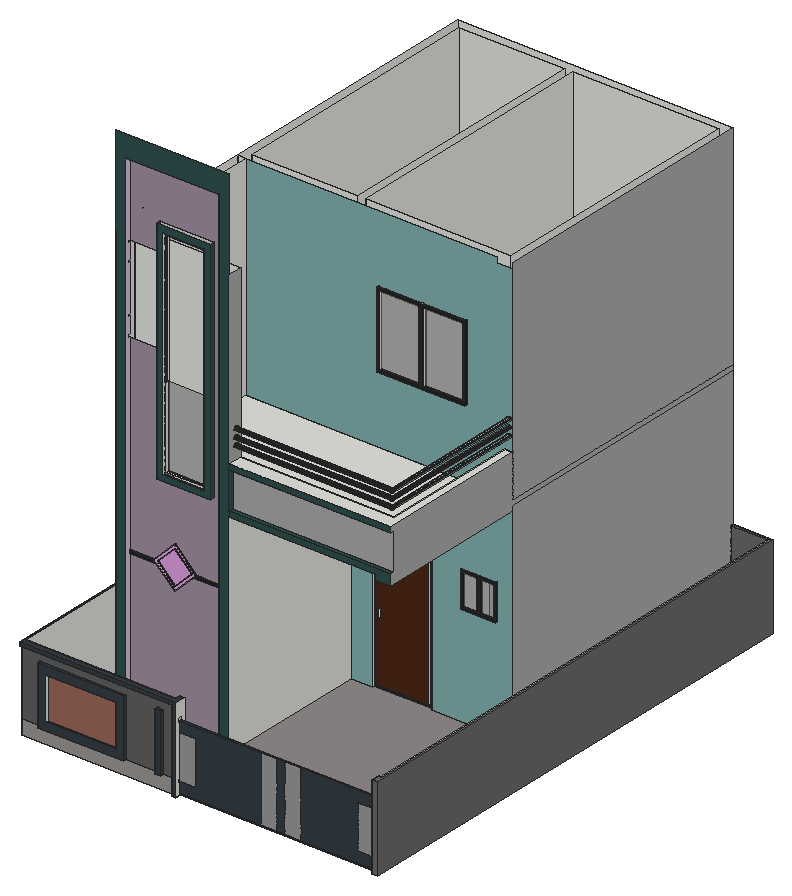
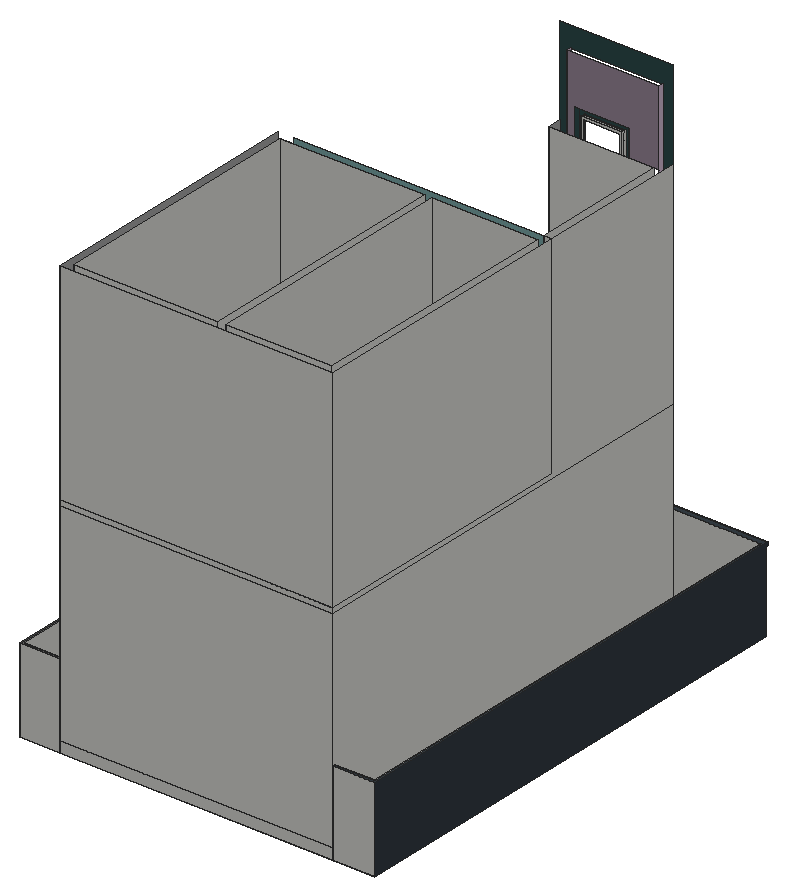
# SketchUp Ruby script. Lengths in inches.
U = 1.inch
M = Sketchup.active_model
def pt(a) = Geom::Point3d.new(a.map { |v| v * U })
def face(e, loops, mat)
  f = e.add_face(loops[0].map { |a| pt(a) })
  loops[1..].each { |l| e.add_face(l.map { |a| pt(a) }).erase! }
  f.material = f.back_material = mat if mat
  f
end
# faces: each face lists its corners as indices into pts; further lists are holes
def faces(e, pts, list, mat = nil) = list.each { |f| face(e, (f[0].is_a?(Array) ? f : [f]).map { |l| l.map { |i| pts[i] } }, mat) }
# xy, xz, yz: faces in a plane at the given z, y or x. An outline is a flat list of corners, or four numbers for a rectangle; further outlines are holes
def ring(l) = l.size == 4 ? [[l[0], l[1]], [l[2], l[1]], [l[2], l[3]], [l[0], l[3]]] : l.each_slice(2).to_a
def flat(e, list, mat, &to3) = list.each { |f| face(e, (f[0].is_a?(Array) ? f : [f]).map { |l| ring(l).map { |u, v| to3.(u, v) } }, mat) }
def xy(e, z, list, mat = nil) = flat(e, list, mat) { |x, y| [x, y, z] }
def xz(e, y, list, mat = nil) = flat(e, list, mat) { |x, z| [x, y, z] }
def yz(e, x, list, mat = nil) = flat(e, list, mat) { |y, z| [x, y, z] }
def lines(e, pts, list) = list.each { |a, b| e.add_line(pt(pts[a]), pt(pts[b])) }
# prism: a flat outline (further loops are holes) pulled along v
def prism(e, loops, v, mat = nil)
  f = face(e, loops, mat); d = Geom::Vector3d.new(v.map { |x| x * U })
  f.pushpull(f.normal.samedirection?(d) ? d.length : -d.length)
end
def box(e, o, s, mat = nil) = prism(e, [[o, [o[0] + s[0], o[1], o[2]], [o[0] + s[0], o[1] + s[1], o[2]], [o[0], o[1] + s[1], o[2]]]], [0, 0, s[2]], mat)
def at(x, y, z, deg = 0) = Geom::Transformation.translation(pt([x, y, z])) * Geom::Transformation.rotation(ORIGIN, Z_AXIS, deg.degrees)
def axes(o, x, y, z) = Geom::Transformation.new([*x, 0, *y, 0, *z, 0, *pt(o).to_a, 1])
def part(name) = M.definitions.add(name)
# library, detail: a bought-in or finely detailed component or shape, given as its bounding box
def library(name, o, s) = part(name).tap { |d| box(d.entities, o, s) }
def detail(e, o, s) = box(e.add_group.entities, o, s)
def put(e, d, t, mat = nil) = e.add_instance(d, t).tap { |i| i.material = mat if mat }
def group(e, t, mat = nil) = e.add_group.tap { |g| g.transformation = t; g.material = mat if mat }.entities
root = M.entities
M.materials.add("[0008_LavenderBlush]").color = [255, 240, 245]
M.materials.add("[0042_Sienna]").color = [76, 39, 21]
M.materials.add("[0078_DarkSlateGray]").color = [47, 79, 79]
M.materials.add("[0089_PaleTurquoise]").color = [129, 175, 175]
M.materials.add("[0090_LightCyan]").color = [165, 188, 188]
M.materials.add("[0111_SlateGray]").color = [53, 61, 68]
M.materials.add("[0118_Thistle]").color = [160, 142, 160]
M.materials.add("[0118_Thistle]1").color = [216, 191, 216]
M.materials.add("[0125_Plum]").color = [221, 160, 221]
M.materials.add("[0132_LightGray]").color = [169, 169, 169]
M.materials.add("[0134_DimGray]").color = [105, 105, 105]
M.materials.add("[0136_Charcoal]").color = [35, 35, 35]
M.materials.add("[Concrete Aggregate Smoke]").color = [154, 150, 148]
M.materials.add("[Granite Dark Gray]").color = [69, 68, 68]
M.materials.add("[Herringbone 4x1]").color = [153, 153, 153]
M.materials.add("[Stone Flagstone Ashlar]").color = [155, 103, 90]
M.materials.add("[Stone Marble]").color = [143, 138, 136]
M.materials.add("[Stone Random Rubble]").color = [96, 96, 96]
M.materials.add("[Translucent Glass Gray]").color = [128, 128, 128]
M.materials["[Translucent Glass Gray]"].alpha = 0.5
xy(root,0,[[172.5,0,172.5,3,0,3,0,560,405,560,405,0,402,0,402,6,177,6,177,0],[399.17,0,402,6]])
xy(root,0.5,[[399.17,6,402,9]])
xy(root,0.5,[[3,6,171,6,171,12,177,12,177,6,399.17,6,399.17,9,402,9,402,557,360,557,360,80,177,80,177,75,48,75,48,557,3,557]],"[Granite Dark Gray]")
xy(root,3.43,[[177,3.29,399.17,5.29]])
xy(root,12,[[57,89,168,248],[57,257,168,551],[177,257,327,551]])
xy(root,12,[[60,75,165,80]],"[0118_Thistle]1")
xy(root,12,[[177,80,360,80,360,248,268.5,248,268.5,250,201.23,250,201.23,248,177,248]],"[Stone Marble]")
xy(root,15.91,[[20.09,0,117.16,3],[153.24,0,159.54,3]],"[0111_SlateGray]")
xy(root,16,[[205.23,248,264.5,250]])
xy(root,24.91,[[29.09,0,108.16,3]])
xy(root,72.91,[[29.09,0,108.16,3]])
xy(root,76.87,[[177,3.29,178.74,5.29]])
xy(root,76.87,[[178.74,3.29,288.09,5.29],[288.09,3.29,297.09,5.29],[297.09,3.29,399.17,5.29]],"[0111_SlateGray]")
xy(root,81.91,[[20.09,0,117.16,3],[153.24,0,159.54,3]],"[0111_SlateGray]")
xy(root,92,[[0,0,172.5,3]])
xy(root,96,[[0,0,177,0,177,12,171,12,171,6,3,6,3,557,48,557,48,560,0,560]],"[0111_SlateGray]")
xy(root,96,[[399.17,0,405,0,405,560,360,560,360,557,402,557,402,9,399.17,9]],"[0134_DimGray]")
xy(root,127.74,[[302.46,246,322.46,248],[322.46,246,342.46,248]],"[0136_Charcoal]")
xy(root,129.74,[[304.46,246,320.46,248],[324.46,246,340.46,248]],"[0136_Charcoal]")
xy(root,164.02,[[205.23,248,264.5,250]])
xy(root,165.74,[[304.46,246,320.46,248],[324.46,246,340.46,248]])
xy(root,167.74,[[302.46,246,322.46,248],[322.46,246,342.46,248]],"[0136_Charcoal]")
xy(root,168.02,[[201.23,248,268.5,250]])
xy(root,172.8,[[60,79,91.75,80]])
xy(root,172.8,[[132.72,79,165,80]],"[0136_Charcoal]")
xy(root,176.05,[[60,79,88.5,80],[135.97,79,165,80]])
xy(root,246,[[342,75,360,248]],"[0078_DarkSlateGray]")
xy(root,252,[[[177,75,342,248],[288.07,123.02,288.86,123.05,289.6,123.29,290.26,123.71,290.79,124.28,291.15,124.98,291.32,125.74,291.29,126.52,291.05,127.27,290.63,127.93,290.06,128.46,289.36,128.82,288.6,128.99,287.82,128.96,287.07,128.72,286.41,128.3,285.88,127.73,285.52,127.03,285.35,126.27,285.38,125.48,285.62,124.74,286.04,124.08,286.61,123.55,287.31,123.1875],[221.7,123.02,222.48,123.05,223.23,123.29,223.89,123.71,224.42,124.28,224.78,124.98,224.95,125.74,224.91,126.52,224.68,127.27,224.26,127.93,223.68,128.46,222.99,128.82,222.22,128.99,221.44,128.96,220.69,128.72,220.03,128.3,219.5,127.73,219.14,127.03,218.97,126.27,219.01,125.48,219.24,124.74,219.66,124.08,220.24,123.55,220.93,123.1875],[221.7,170.7,222.48,170.74,223.23,170.97,223.89,171.39,224.42,171.97,224.78,172.67,224.95,173.43,224.91,174.21,224.68,174.96,224.26,175.62,223.68,176.15,222.99,176.51,222.22,176.68,221.44,176.65,220.69,176.41,220.03,175.99,219.5,175.41,219.14,174.72,218.97,173.95,219.01,173.17,219.24,172.42,219.66,171.76,220.24,171.23,220.93,170.875],[285.2,170.7,285.98,170.74,286.73,170.97,287.39,171.39,287.92,171.97,288.28,172.67,288.45,173.43,288.41,174.21,288.18,174.96,287.76,175.62,287.18,176.15,286.49,176.51,285.72,176.68,284.94,176.65,284.19,176.41,283.53,175.99,283,175.41,282.64,174.72,282.47,173.95,282.51,173.17,282.74,172.42,283.16,171.76,283.74,171.23,284.43,170.875]],[221.7,123.02,220.93,123.1875,220.24,123.55,219.66,124.08,219.24,124.74,219.01,125.48,218.97,126.27,219.14,127.03,219.5,127.73,220.03,128.3,220.69,128.72,221.44,128.96,222.22,128.99,222.99,128.82,223.68,128.46,224.26,127.93,224.68,127.27,224.91,126.52,224.95,125.74,224.78,124.98,224.42,124.28,223.89,123.71,223.23,123.29,222.48,123.05],[288.07,123.02,287.31,123.1875,286.61,123.55,286.04,124.08,285.62,124.74,285.38,125.48,285.35,126.27,285.52,127.03,285.88,127.73,286.41,128.3,287.07,128.72,287.82,128.96,288.6,128.99,289.36,128.82,290.06,128.46,290.63,127.93,291.05,127.27,291.29,126.52,291.32,125.74,291.15,124.98,290.79,124.28,290.26,123.71,289.6,123.29,288.86,123.05],[221.7,170.7,220.93,170.875,220.24,171.23,219.66,171.76,219.24,172.42,219.01,173.17,218.97,173.95,219.14,174.72,219.5,175.41,220.03,175.99,220.69,176.41,221.44,176.65,222.22,176.68,222.99,176.51,223.68,176.15,224.26,175.62,224.68,174.96,224.91,174.21,224.95,173.43,224.78,172.67,224.42,171.97,223.89,171.39,223.23,170.97,222.48,170.74],[285.2,170.7,284.43,170.875,283.74,171.23,283.16,171.76,282.74,172.42,282.51,173.17,282.47,173.95,282.64,174.72,283,175.41,283.53,175.99,284.19,176.41,284.94,176.65,285.72,176.68,286.49,176.51,287.18,176.15,287.76,175.62,288.18,174.96,288.41,174.21,288.45,173.43,288.28,172.67,287.92,171.97,287.39,171.39,286.73,170.97,285.98,170.74]])
xy(root,258,[[57,91,351,248],[[48,248,360,560],[186,257,351,551],[57,257,177,551]],[57,257,177,551],[186,257,351,551]])
xy(root,258,[[177,75,360,80]],"[0078_DarkSlateGray]")
xy(root,261.51,[[94.88,75,155.82,80]],"[0078_DarkSlateGray]")
xy(root,268.7,[[102.07,75,148.63,77],[102.07,77,148.63,80]])
xy(root,270.7,[[104.07,77,146.63,80]])
xy(root,300,[[177,75,360,80]],"[0078_DarkSlateGray]")
xy(root,306,[[177,75,360,75,360,248,351,248,351,91,177,91]])
xy(root,335.48,[[257.89,248,259.89,250]])
xy(root,335.48,[[207.99,246,257.89,248],[257.89,246,259.89,248],[259.89,246,307.8,248]],"[0136_Charcoal]")
xy(root,338.48,[[210.99,246,254.89,248],[260.89,246,304.8,248]])
xz(root,0,[[172.5,0,177,0,177,96,0,96,0,92,172.5,92],[[20.09,15.91,117.16,81.91],[29.09,24.91,108.16,72.91]],[153.24,15.91,159.54,81.91]],"[0111_SlateGray]")
xz(root,0,[[399.17,0,405,96]],"[0134_DimGray]")
xz(root,3,[[0,0,172.5,15.91]],"[Concrete Aggregate Smoke]")
xz(root,3,[[29.09,24.91,108.16,72.91]],"[Stone Flagstone Ashlar]")
xz(root,3,[[0,15.91,20.09,15.91,20.09,81.91,117.16,81.91,117.16,15.91,153.24,15.91,153.24,81.91,159.54,81.91,159.54,15.91,172.5,15.91,172.5,92,0,92]],"[Stone Random Rubble]")
xz(root,3.29,[[177,3.43,270.09,3.43,270.09,76.87,177,76.87,177,64.74,196.5,64.74,196.5,15.12,177,15.12],[288.09,3.43,297.09,76.87],[315.09,3.43,399.17,3.43,399.17,15.12,379.67,15.12,379.67,64.74,399.17,64.74,399.17,76.87,315.09,76.87]],"[0111_SlateGray]")
xz(root,3.29,[[270.09,3.43,288.09,76.87],[297.09,3.43,315.09,76.87],[177,15.12,196.5,64.74],[379.67,15.12,399.17,64.74]],"[Herringbone 4x1]")
xz(root,5.29,[[177,3.43,288.09,76.87],[288.09,3.43,297.09,76.87],[297.09,3.43,399.17,76.87]],"[0111_SlateGray]")
xz(root,6,[[177,0,399.17,0.5],[399.17,0,402,0.5],[3,0.5,171,96]])
xz(root,9,[[399.17,0.5,402,96]])
xz(root,12,[[171,0.5,177,96]])
xz(root,75,[[[48,0.5,177,600],[60,12,165,576]],[342,246,360,246,360,258,177,258,177,252,342,252],[[94.88,261.51,155.82,521.33],[102.07,268.7,148.63,514.14]],[177,300,360,306]],"[0078_DarkSlateGray]")
xz(root,77,[[[102.07,268.7,148.63,514.14],[104.07,270.7,146.63,512.14]]])
xz(root,79,[[[112.23,152.32,132.72,172.8,135.97,176.05,112.23,199.78,88.5,176.05],[112.23,156.56,92.74,176.05,112.23,195.54,131.72,176.05]]],"[0125_Plum]")
xz(root,79,[[60,172.8,91.75,172.8,88.5,176.05,60,176.05],[132.72,172.8,165,172.8,165,176.05,135.97,176.05]],"[0136_Charcoal]")
xz(root,80,[[[102.07,268.7,148.63,514.14],[104.07,270.7,146.63,512.14]]])
xz(root,80,[[60,12,165,12,165,172.8,132.72,172.8,112.23,152.32,91.75,172.8,60,172.8],[[60,176.05,88.5,176.05,112.23,199.78,135.97,176.05,165,176.05,165,576,60,576,60,490.5,94.88,490.5,94.88,521.33,155.82,521.33,155.82,261.51,94.88,261.51,94.88,391.54,60,391.54],[73.93,526.2,73.97,526.61,73.91,526.44,73.88,526.35,73.91,526.44,73.97,526.61,74.05,527.02,74.17,527.41,74.33,527.79,74.41,527.93,74.49,528.17,75.27,531.36,75.77,534.61,76,537.89,75.99,538.9375,75.9,539.34,75.85,539.75,75.85,540.16,75.88,540.57,75.96,540.96,75.96,541.17,75.63,544.44,75.07,547.51,74.27,550.51,74.15,550.9,74.08,551.22,74.0625,551.31,74.02,551.72,74.02,552.13,74.07,552.54,74.15,552.9375,74.28,553.33,74.45,553.71,74.65,554.0625,74.89,554.4,75.17,554.7,75.47,554.98,75.59,554.59,75.68,554.1875,75.72,553.78,75.72,553.37,75.67,552.96,75.59,552.55,75.46,552.16,75.29,551.79,75.09,551.43,74.85,551.1,74.58,550.79,74.27,550.51,75.07,547.51,75.63,544.44,75.96,541.17,75.96,540.96,75.96,540.97,76.08,541.36,76.24,541.74,76.44,542.1,76.68,542.44,76.94,542.75,77.24,543.03,77.57,543.28,77.66,542.88,77.71,542.47,77.71,542.0625,77.68,541.65,77.6,541.25,77.48,540.86,77.32,540.48,77.12,540.12,76.88,539.78,76.61,539.47,76.31,539.1875,75.99,538.9375,76,537.89,75.77,534.61,75.27,531.36,74.49,528.17,74.41,527.93,74.53,528.15,74.76,528.48,75.03,528.79,75.33,529.08,75.66,529.32,76.01,529.54,76.38,529.71,76.77,529.85,76.73,529.44,76.65,529.04,76.53,528.65,76.37,528.27,76.17,527.91,75.93,527.57,75.66,527.26,75.36,526.98,75.04,526.73,74.6875,526.52,74.32,526.34],[74.27,550.51,73.87,550.6,73.48,550.73,73.11,550.9,72.75,551.11,72.42,551.35,72.11,551.625,71.84,551.93,71.59,552.26,71.39,552.62,71.22,552.99,71.09,553.38,71,553.78,71.4,553.69,71.79,553.57,72.17,553.4,72.52,553.19,72.86,552.95,73.16,552.67,73.4375,552.37,73.68,552.03,73.82,551.8,73.23,553.45,71.96,556.29,70.59,558.8,70.25,559.04,69.95,559.32,69.67,559.62,69.43,559.95,69.22,560.31,69.05,560.68,68.92,561.07,68.83,561.47,68.78,561.88,68.77,562.29,68.8125,562.7,68.89,563.11,69.22,562.86,69.53,562.59,69.81,562.29,70.05,561.95,70.26,561.6,70.43,561.23,70.56,560.84,70.65,560.43,70.7,560.03,70.7,559.62,70.66,559.21,70.59,558.8,71.96,556.29,73.23,553.45,73.82,551.8,73.88,551.68,74.05,551.3,74.08,551.22,74.18,550.91],[75.99,538.9375,75.59,539.03,75.2,539.15,74.82,539.32,74.47,539.53,74.13,539.77,73.83,540.05,73.55,540.35,73.3125,540.6875,73.1,541.04,72.9375,541.42,72.81,541.81,72.72,542.21,73.12,542.12,73.51,541.99,73.88,541.82,74.24,541.61,74.57,541.37,74.88,541.1,75.15,540.79,75.39,540.46,75.53,540.22],[73.86,526.09,73.8,526.12,73.58,526.24,73.23,526.47,72.91,526.73,72.625,527.02,72.37,527.34,72.14,527.68,71.96,528.05,71.81,528.43,71.7,528.83,71.63,529.23,71.61,529.65,71.63,530.06,71.99,529.87,72.34,529.64,72.65,529.38,72.94,529.09,73.2,528.77,73.43,528.42,73.61,528.06,73.76,527.67,73.83,527.41,73.91,526.44,73.93,526.2]]],"[0118_Thistle]")
xz(root,80,[[112.23,156.56,131.72,176.05,112.23,195.54,92.74,176.05]],"[0125_Plum]")
xz(root,80,[[177,258,360,300]],"[0132_LightGray]")
xz(root,80,[[177,0.5,360,12]],"[Stone Marble]")
xz(root,80,[[104.07,270.7,146.63,362.14]],"[Translucent Glass Gray]")
xz(root,89,[[57,12,168,252]])
xz(root,91,[[57,258,177,498],[177,258,351,306]])
xz(root,246,[[[302.46,127.74,322.46,167.74],[304.46,129.74,320.46,165.74]],[[322.46,127.74,342.46,167.74],[324.46,129.74,340.46,165.74]],[[207.99,335.48,257.89,421.73],[210.99,338.48,254.89,418.73]],[[257.89,335.48,307.8,421.73],[260.89,338.48,304.8,418.73]]],"[0136_Charcoal]")
xz(root,248,[[57,12,168,252],[48,258,57,498],[351,258,360,306],[[207.99,335.48,257.89,421.73],[210.99,338.48,254.89,418.73]],[[257.89,335.48,307.8,421.73],[260.89,338.48,304.8,418.73]]])
xz(root,248,[[207.39,84.08,210.14,95.58]],"[0008_LavenderBlush]")
xz(root,248,[[[205.23,16,264.5,164.02],[207.39,84.08,210.14,95.58]]],"[0042_Sienna]")
xz(root,248,[[[177,12,201.23,12,201.23,168.02,268.5,168.02,268.5,12,360,12,360,246,342,246,342,252,177,252],[302.46,127.74,342.46,167.74]],[[57,258,351,258,351,306,360,306,360,492,342,492,342,498,57,498],[207.99,335.48,307.8,421.73],[356.1,319.56,355.58,319.625,355.1,319.83,354.6875,320.14,354.37,320.56,354.17,321.04,354.1,321.56,354.17,322.08,354.37,322.56,354.6875,322.97,355.1,323.29,355.58,323.49,356.1,323.56,356.62,323.49,357.1,323.29,357.52,322.97,357.83,322.56,358.03,322.08,358.1,321.56,358.03,321.04,357.83,320.56,357.52,320.14,357.1,319.83,356.62,319.625],[356.1,336.75,355.58,336.8125,355.1,337.01,354.6875,337.33,354.37,337.75,354.17,338.23,354.1,338.75,354.17,339.26,354.37,339.75,354.6875,340.16,355.1,340.48,355.58,340.68,356.1,340.75,356.62,340.68,357.1,340.48,357.52,340.16,357.83,339.75,358.03,339.26,358.1,338.75,358.03,338.23,357.83,337.75,357.52,337.33,357.1,337.01,356.62,336.8125]]],"[0089_PaleTurquoise]")
xz(root,248,[[304.46,129.74,320.46,165.74],[324.46,129.74,340.46,165.74],[210.99,338.48,254.89,418.73],[260.89,338.48,304.8,418.73]],"[Translucent Glass Gray]")
xz(root,250,[[257.89,335.48,259.89,421.73]])
xz(root,250,[[[201.23,12,268.5,168.02],[205.23,16,264.5,164.02]]],"[0136_Charcoal]")
xz(root,257,[[57,12,168,252],[177,12,327,252],[57,258,177,498],[186,258,351,498]])
xz(root,551,[[57,12,168,252],[177,12,327,252],[57,258,177,498],[186,258,351,498]])
xz(root,557,[[3,0.5,48,96]])
xz(root,557,[[360,0.5,402,96]],"[0134_DimGray]")
xz(root,560,[[0,0,48,96],[48,0,360,12],[360,0,405,96],[48,12,360,252],[48,252,360,258],
  [48,258,360,498]])
yz(root,0,[[3,0,3,92,0,92,0,96,560,96,560,0]],"[0111_SlateGray]")
yz(root,3,[[6,0.5,557,96]])
yz(root,20.09,[[0,15.91,3,81.91]],"[0111_SlateGray]")
yz(root,29.09,[[0,24.91,3,72.91]])
yz(root,48,[[75,0,75,0.5,557,0.5,557,96,560,96,560,0],[75,0.5,557,12],[75,12,75,252,560,252,560,96,557,96,557,12],[75,252,75,498,248,498,248,258,560,258,560,252],[248,258,560,498]])
yz(root,57,[[89,12,248,252],[257,12,551,252],[91,258,248,498],[257,258,551,498]])
yz(root,60,[[75,12,80,12,80,172.8,79,172.8,79,176.05,80,176.05,80,391.54,78,391.54,78,394.13,80,394.13,80,412.82,78,412.82,78,415.1875,80,415.1875,80,467.57,78,467.57,78,469.9375,80,469.9375,80,488.13,78,488.13,78,490.5,80,490.5,80,576,75,576]],"[0118_Thistle]1")
yz(root,94.88,[[75,261.51,75,521.33,80,521.33,80,490.5,78,490.5,78,488.13,80,488.13,80,469.9375,78,469.9375,78,467.57,80,467.57,80,415.1875,78,415.1875,78,412.82,80,412.82,80,394.13,78,394.13,78,391.54,80,391.54,80,261.51]],"[0078_DarkSlateGray]")
yz(root,102.07,[[75,268.7,77,514.14],[77,268.7,80,514.14]])
yz(root,104.07,[[77,270.7,80,362.14]])
yz(root,108.16,[[0,24.91,3,72.91]])
yz(root,117.16,[[0,15.91,3,81.91]],"[0111_SlateGray]")
yz(root,146.63,[[77,270.7,80,362.14]])
yz(root,148.63,[[75,268.7,77,514.14],[77,268.7,80,514.14]])
yz(root,153.24,[[0,15.91,3,81.91]],"[0111_SlateGray]")
yz(root,155.82,[[75,261.51,80,521.33]],"[0078_DarkSlateGray]")
yz(root,159.54,[[0,15.91,3,81.91]],"[0111_SlateGray]")
yz(root,165,[[75,12,75,576,80,576,80,176.05,79,176.05,79,172.8,80,172.8,80,12]],"[0118_Thistle]1")
yz(root,168,[[89,12,248,252],[257,12,551,252]])
yz(root,171,[[6,0.5,12,96]])
yz(root,172.5,[[0,0,3,15.91],[0,15.91,3,92]])
yz(root,177,[[0,0,6,0.5],[[0,0.5,12,96],[5.29,12.43,4.51,12.53,3.79,12.83,3.29,13.22,3.17,13.31,2.69,13.93,2.39,14.65,2.29,15.43,2.39,16.21,2.69,16.93,3.17,17.55,3.29,17.65,3.29,73.87,5.29,73.87,4.51,73.97,3.79,74.27,3.29,74.65,3.17,74.75,2.69,75.37,2.39,76.09,2.29,76.87,2.39,77.64,2.69,78.37,3.17,78.99,3.79,79.47,4.51,79.77,5.29,79.87,6.07,79.77,6.79,79.47,7.41,78.99,7.89,78.37,8.1875,77.64,8.29,76.87,8.1875,76.09,7.89,75.37,7.41,74.75,6.79,74.27,6.07,73.97,5.29,73.87,5.29,18.43,6.07,18.33,6.79,18.03,7.41,17.55,7.89,16.93,8.1875,16.21,8.29,15.43,8.1875,14.65,7.89,13.93,7.41,13.31,6.79,12.83,6.07,12.53]],[75,0.5,80,0.5,80,12,248,12,248,252,75,252],[3.29,3.43,3.29,13.22,3.79,12.83,4.51,12.53,5.29,12.43,5.29,3.43],[257,12,551,252],
  [5.29,12.43,4.51,12.53,3.79,12.83,3.29,13.22,3.29,15.43,5.29,15.43],[5.29,12.43,6.07,12.53,6.79,12.83,7.41,13.31,7.89,13.93,8.1875,14.65,8.29,15.43,8.1875,16.21,7.89,16.93,7.41,17.55,6.79,18.03,6.07,18.33,5.29,18.43],[3.29,13.22,3.29,17.65,3.17,17.55,2.69,16.93,2.39,16.21,2.29,15.43,2.39,14.65,2.69,13.93,3.17,13.31],[3.29,15.43,3.29,17.65,3.79,18.03,4.51,18.33,5.29,18.43,5.29,15.43],[3.29,17.65,3.79,18.03,4.51,18.33,5.29,18.43,3.29,18.43],
  [3.29,18.43,5.29,73.87],[5.29,73.87,6.07,73.97,6.79,74.27,7.41,74.75,7.89,75.37,8.1875,76.09,8.29,76.87,8.1875,77.64,7.89,78.37,7.41,78.99,6.79,79.47,6.07,79.77,5.29,79.87,4.51,79.77,3.79,79.47,3.17,78.99,2.69,78.37,2.39,77.64,2.29,76.87,2.39,76.09,2.69,75.37,3.17,74.75,3.29,74.65,3.29,76.87,5.29,76.87],[3.29,73.87,3.29,74.65,3.79,74.27,4.51,73.97,5.29,73.87],[5.29,73.87,4.51,73.97,3.79,74.27,3.29,74.65,3.29,76.87,5.29,76.87],[257,258,551,498],
  [83,319.56,82.48,319.625,82,319.83,81.59,320.14,81.27,320.56,81.07,321.04,81,321.56,81.07,322.08,81.27,322.56,81.59,322.97,82,323.29,82.48,323.49,83,323.56,83.52,323.49,84,323.29,84.41,322.97,84.73,322.56,84.93,322.08,85,321.56,84.93,321.04,84.73,320.56,84.41,320.14,84,319.83,83.52,319.625],[82.98,328.02,83.49,328.09,83.98,328.29,84.39,328.61,84.71,329.02,84.91,329.51,84.98,330.02,84.91,330.54,84.71,331.02,84.39,331.4375,83.98,331.76,83.49,331.96,82.98,332.02,82.46,331.96,81.98,331.76,81.5625,331.4375,81.24,331.02,81.04,330.54,80.98,330.02,81.04,329.51,81.24,329.02,81.5625,328.61,81.98,328.29,82.46,328.09],[83,336.75,82.48,336.8125,82,337.01,81.59,337.33,81.27,337.75,81.07,338.23,81,338.75,81.07,339.26,81.27,339.75,81.59,340.16,82,340.48,82.48,340.68,83,340.75,83.52,340.68,84,340.48,84.41,340.16,84.73,339.75,84.93,339.26,85,338.75,84.93,338.23,84.73,337.75,84.41,337.33,84,337.01,83.52,336.8125]])
yz(root,177,[[75,258,80,300]],"[0078_DarkSlateGray]")
yz(root,177,[[[75,306,91,498],[83,319.56,82.48,319.625,82,319.83,81.59,320.14,81.27,320.56,81.07,321.04,81,321.56,81.07,322.08,81.27,322.56,81.59,322.97,82,323.29,82.48,323.49,83,323.56,83.52,323.49,84,323.29,84.41,322.97,84.73,322.56,84.93,322.08,85,321.56,84.93,321.04,84.73,320.56,84.41,320.14,84,319.83,83.52,319.625],[82.98,328.02,82.46,328.09,81.98,328.29,81.5625,328.61,81.24,329.02,81.04,329.51,80.98,330.02,81.04,330.54,81.24,331.02,81.5625,331.4375,81.98,331.76,82.46,331.96,82.98,332.02,83.49,331.96,83.98,331.76,84.39,331.4375,84.71,331.02,84.91,330.54,84.98,330.02,84.91,329.51,84.71,329.02,84.39,328.61,83.98,328.29,83.49,328.09],[83,336.75,82.48,336.8125,82,337.01,81.59,337.33,81.27,337.75,81.07,338.23,81,338.75,81.07,339.26,81.27,339.75,81.59,340.16,82,340.48,82.48,340.68,83,340.75,83.52,340.68,84,340.48,84.41,340.16,84.73,339.75,84.93,339.26,85,338.75,84.93,338.23,84.73,337.75,84.41,337.33,84,337.01,83.52,336.8125]]],"[0132_LightGray]")
yz(root,186,[[257,258,551,498]])
yz(root,201.23,[[248,12,250,168.02]])
yz(root,205.23,[[248,16,250,164.02]])
yz(root,207.99,[[246,335.48,248,421.73]],"[0136_Charcoal]")
yz(root,210.99,[[246,338.48,248,418.73]])
yz(root,254.89,[[246,338.48,248,418.73]])
yz(root,257.89,[[246,335.48,248,421.73],[248,335.48,250,421.73]])
yz(root,260.89,[[246,338.48,248,418.73]])
yz(root,264.5,[[248,16,250,164.02]])
yz(root,268.5,[[248,12,250,168.02]])
yz(root,302.46,[[246,127.74,248,167.74]],"[0136_Charcoal]")
yz(root,304.46,[[246,129.74,248,165.74]],"[0136_Charcoal]")
yz(root,304.8,[[246,338.48,248,418.73]])
yz(root,307.8,[[246,335.48,248,421.73]],"[0136_Charcoal]")
yz(root,320.46,[[246,129.74,248,165.74]],"[0136_Charcoal]")
yz(root,324.46,[[246,129.74,248,165.74]],"[0136_Charcoal]")
yz(root,327,[[257,12,551,252]])
yz(root,340.46,[[246,129.74,248,165.74]],"[0136_Charcoal]")
yz(root,342,[[75,246,248,252]],"[0078_DarkSlateGray]")
yz(root,342.46,[[246,127.74,248,167.74]],"[0136_Charcoal]")
yz(root,351,[[91,258,248,306],[257,258,551,498]])
yz(root,360,[[80,0,560,0,560,96,557,96,557,0.5,80,0.5],[80,0.5,557,12]])
yz(root,360,[[248,12,557,12,557,96,560,96,560,252,248,252],[75,246,248,246,248,252,560,252,560,258,248,258,248,306,75,306,75,300,80,300,80,258,75,258],[248,258,560,498]],"[0132_LightGray]")
yz(root,399.17,[[[0,0,0,96,9,96,9,0.5,6,0.5,6,0],[5.29,12.43,6.07,12.53,6.79,12.83,7.41,13.31,7.89,13.93,8.1875,14.65,8.29,15.43,8.1875,16.21,7.89,16.93,7.41,17.55,6.79,18.03,6.07,18.33,5.29,18.43,5.29,73.74,6.07,73.85,6.79,74.15,7.41,74.62,7.89,75.24,8.1875,75.97,8.29,76.74,8.1875,77.52,7.89,78.24,7.41,78.86,6.79,79.34,6.07,79.64,5.29,79.74,4.51,79.64,3.79,79.34,3.17,78.86,2.69,78.24,2.39,77.52,2.29,76.74,2.39,75.97,2.69,75.24,3.17,74.62,3.29,74.53,3.79,74.15,4.51,73.85,5.29,73.74,3.29,73.74,3.29,17.65,3.17,17.55,2.69,16.93,2.39,16.21,2.29,15.43,2.39,14.65,2.69,13.93,3.17,13.31,3.29,13.22,3.79,12.83,4.51,12.53]],[3.29,3.43,5.29,3.43,5.29,12.43,4.51,12.53,3.79,12.83,3.29,13.22],[5.29,12.43,5.29,15.43,3.29,15.43,3.29,13.22,3.79,12.83,4.51,12.53],[5.29,12.43,5.29,18.43,6.07,18.33,6.79,18.03,7.41,17.55,7.89,16.93,8.1875,16.21,8.29,15.43,8.1875,14.65,7.89,13.93,7.41,13.31,6.79,12.83,6.07,12.53],[3.29,13.22,3.17,13.31,2.69,13.93,2.39,14.65,2.29,15.43,2.39,16.21,2.69,16.93,3.17,17.55,3.29,17.65],
  [3.29,15.43,5.29,15.43,5.29,18.43,4.51,18.33,3.79,18.03,3.29,17.65],[3.29,17.65,3.29,18.43,5.29,18.43,4.51,18.33,3.79,18.03],[3.29,18.43,5.29,73.74],[5.29,73.74,5.29,76.87,3.29,76.87,3.29,74.53,3.17,74.62,2.69,75.24,2.39,75.97,2.29,76.74,2.39,77.52,2.69,78.24,3.17,78.86,3.79,79.34,4.51,79.64,5.29,79.74,6.07,79.64,6.79,79.34,7.41,78.86,7.89,78.24,8.1875,77.52,8.29,76.74,8.1875,75.97,7.89,75.24,7.41,74.62,6.79,74.15,6.07,73.85],[3.29,73.74,5.29,73.74,4.51,73.85,3.79,74.15,3.29,74.53],
  [5.29,73.74,5.29,76.87,3.29,76.87,3.29,74.53,3.79,74.15,4.51,73.85]])
yz(root,402,[[9,0.5,557,96]])
yz(root,405,[[0,0,560,96]],"[0134_DimGray]")
p = [[91.75,80,172.8],[112.23,80,152.32],[112.23,79,152.32],[91.75,79,172.8],[132.72,80,172.8],[132.72,79,172.8],
  [92.74,79,176.05],[112.23,79,156.56],[112.23,80,156.56],[92.74,80,176.05],[131.72,79,176.05],[131.72,80,176.05],
  [112.23,80,199.78],[88.5,80,176.05],[88.5,79,176.05],[112.23,79,199.78],[112.23,80,195.54],[112.23,79,195.54],
  [135.97,80,176.05],[135.97,79,176.05],[177,82,319.83],[177,82.48,319.625],[356.62,82.48,319.625],[357.1,82,319.83],
  [356.62,248,319.625],[357.1,248,319.83],[177,83,319.56],[356.1,83,319.56],[356.1,248,319.56],[177,83.52,319.625],
  [355.58,83.52,319.625],[355.58,248,319.625],[177,84,319.83],[355.1,84,319.83],[355.1,248,319.83],[177,81.59,320.14],
  [357.52,81.59,320.14],[357.52,248,320.14],[177,84.41,320.14],[354.6875,84.41,320.14],[354.6875,248,320.14],[177,81.27,320.56],
  [357.83,81.27,320.56],[357.83,248,320.56],[177,84.73,320.56],[354.37,84.73,320.56],[354.37,248,320.56],[177,81.07,321.04],
  [358.03,81.07,321.04],[358.03,248,321.04],[177,84.93,321.04],[354.17,84.93,321.04],[354.17,248,321.04],[177,81,321.56],
  [358.1,81,321.56],[358.1,248,321.56],[177,85,321.56],[354.1,85,321.56],[354.1,248,321.56],[177,81.07,322.08],
  [358.03,81.07,322.08],[358.03,248,322.08],[177,84.93,322.08],[354.17,84.93,322.08],[354.17,248,322.08],[177,81.27,322.56],
  [357.83,81.27,322.56],[357.83,248,322.56],[177,84.73,322.56],[354.37,84.73,322.56],[354.37,248,322.56],[177,81.59,322.97],
  [357.52,81.59,322.97],[357.52,248,322.97],[177,84.41,322.97],[354.6875,84.41,322.97],[354.6875,248,322.97],[177,82,323.29],
  [357.1,82,323.29],[357.1,248,323.29],[177,84,323.29],[355.1,84,323.29],[355.1,248,323.29],[177,82.48,323.49],
  [356.62,82.48,323.49],[356.62,248,323.49],[177,83.52,323.49],[355.58,83.52,323.49],[355.58,248,323.49],[177,83,323.56],
  [356.1,83,323.56],[356.1,248,323.56],[177,82.46,328.09],[177,82.98,328.02],[356.1,82.98,328.02],[356.62,82.46,328.09],
  [356.1,83,328.02],[356.1,247.98,328.02],[356.62,247.98,328.09],[177,83.49,328.09],[355.58,83.49,328.09],[355.58,247.98,328.09],
  [177,81.98,328.29],[357.1,81.98,328.29],[357.1,247.98,328.29],[177,83.98,328.29],[355.1,83.98,328.29],[355.1,247.98,328.29],
  [177,81.5625,328.61],[357.52,81.5625,328.61],[357.52,247.98,328.61],[177,84.39,328.61],[354.6875,84.39,328.61],[354.6875,247.98,328.61],
  [177,81.24,329.02],[357.83,81.24,329.02],[357.83,247.98,329.02],[177,84.71,329.02],[354.37,84.71,329.02],[354.37,247.98,329.02],
  [177,81.04,329.51],[358.03,81.04,329.51],[358.03,247.98,329.51],[177,84.91,329.51],[354.17,84.91,329.51],[354.17,247.98,329.51],
  [177,80.98,330.02],[358.1,80.98,330.02],[358.1,247.98,330.02],[177,84.98,330.02],[354.1,84.98,330.02],[354.1,247.98,330.02],
  [177,81.04,330.54],[358.03,81.04,330.54],[358.03,247.98,330.54],[177,84.91,330.54],[354.17,84.91,330.54],[354.17,247.98,330.54],
  [177,81.24,331.02],[357.83,81.24,331.02],[357.83,247.98,331.02],[177,84.71,331.02],[354.37,84.71,331.02],[354.37,247.98,331.02],
  [177,81.5625,331.4375],[357.52,81.5625,331.4375],[357.52,247.98,331.4375],[177,84.39,331.4375],[354.6875,84.39,331.4375],[354.6875,247.98,331.4375],
  [177,81.98,331.76],[357.1,81.98,331.76],[357.1,247.98,331.76],[177,83.98,331.76],[355.1,83.98,331.76],[355.1,247.98,331.76],
  [177,82.46,331.96],[356.62,82.46,331.96],[356.62,247.98,331.96],[177,83.49,331.96],[355.58,83.49,331.96],[355.58,247.98,331.96],
  [177,82.98,332.02],[356.1,82.98,332.02],[356.1,247.98,332.02],[356.1,83,332.02],[177,82.48,336.8125],[177,83,336.75],
  [356.1,83,336.75],[356.62,82.48,336.8125],[356.1,248,336.75],[356.62,248,336.8125],[177,83.52,336.8125],[355.58,83.52,336.8125],
  [355.58,248,336.8125],[177,82,337.01],[357.1,82,337.01],[357.1,248,337.01],[177,84,337.01],[355.1,84,337.01],
  [355.1,248,337.01],[177,81.59,337.33],[357.52,81.59,337.33],[357.52,248,337.33],[177,84.41,337.33],[354.6875,84.41,337.33],
  [354.6875,248,337.33],[177,81.27,337.75],[357.83,81.27,337.75],[357.83,248,337.75],[177,84.73,337.75],[354.37,84.73,337.75],
  [354.37,248,337.75],[177,81.07,338.23],[358.03,81.07,338.23],[358.03,248,338.23],[177,84.93,338.23],[354.17,84.93,338.23],
  [354.17,248,338.23],[177,81,338.75],[358.1,81,338.75],[358.1,248,338.75],[177,85,338.75],[354.1,85,338.75],
  [354.1,248,338.75],[177,81.07,339.26],[358.03,81.07,339.26],[358.03,248,339.26],[177,84.93,339.26],[354.17,84.93,339.26],
  [354.17,248,339.26],[177,81.27,339.75],[357.83,81.27,339.75],[357.83,248,339.75],[177,84.73,339.75],[354.37,84.73,339.75],
  [354.37,248,339.75],[177,81.59,340.16],[357.52,81.59,340.16],[357.52,248,340.16],[177,84.41,340.16],[354.6875,84.41,340.16],
  [354.6875,248,340.16],[177,82,340.48],[357.1,82,340.48],[357.1,248,340.48],[177,84,340.48],[355.1,84,340.48],
  [355.1,248,340.48],[177,82.48,340.68],[356.62,82.48,340.68],[356.62,248,340.68],[177,83.52,340.68],[355.58,83.52,340.68],
  [355.58,248,340.68],[177,83,340.75],[356.1,83,340.75],[356.1,248,340.75],[360,80,0],[360,75,0],
  [177,83,321.56],[356.1,83,321.56],[177,83,338.75],[356.1,83,338.75],[356.1,248,338.75],[356.1,82.98,330.02],
  [356.1,83,330.02],[356.1,248,330.02],[356.1,248,321.56],[177,82.98,330.02]]
faces(root,p,[[0,1,2,3],[1,4,5,2],[12,13,14,15],[18,12,15,19]],"[0125_Plum]")
faces(root,p,[[6,7,8,9],[10,11,8,7],[9,16,17,6],[16,11,10,17]],"[0136_Charcoal]")
faces(root,p,[[20,21,22,23],[23,22,24,25],[21,26,27,22],[22,27,28,24],[26,29,30,27],[27,30,31,28],[29,32,33,30],[30,33,34,31],
  [35,20,23,36],[36,23,25,37],[32,38,39,33],[33,39,40,34],[41,35,36,42],[42,36,37,43],[38,44,45,39],[39,45,46,40],
  [47,41,42,48],[48,42,43,49],[44,50,51,45],[45,51,52,46],[53,47,48,54],[54,48,49,55],[50,56,57,51],[51,57,58,52],
  [59,53,54,60],[60,54,55,61],[56,62,63,57],[57,63,64,58],[65,59,60,66],[66,60,61,67],[62,68,69,63],[63,69,70,64],
  [71,65,66,72],[72,66,67,73],[68,74,75,69],[69,75,76,70],[77,71,72,78],[78,72,73,79],[74,80,81,75],[75,81,82,76],
  [83,77,78,84],[84,78,79,85],[80,86,87,81],[81,87,88,82],[89,83,84,90],[90,84,85,91],[86,89,90,87],[87,90,91,88],
  [92,93,94,95],[95,94,96,97,98],[93,99,100,94],[94,100,101,97,96],[102,92,95,103],[103,95,98,104],[99,105,106,100],[100,106,107,101],
  [108,102,103,109],[109,103,104,110],[105,111,112,106],[106,112,113,107],[114,108,109,115],[115,109,110,116],[111,117,118,112],[112,118,119,113],
  [120,114,115,121],[121,115,116,122],[117,123,124,118],[118,124,125,119],[126,120,121,127],[127,121,122,128],[123,129,130,124],[124,130,131,125],
  [132,126,127,133],[133,127,128,134],[129,135,136,130],[130,136,137,131],[138,132,133,139],[139,133,134,140],[135,141,142,136],[136,142,143,137],
  [144,138,139,145],[145,139,140,146],[141,147,148,142],[142,148,149,143],[150,144,145,151],[151,145,146,152],[147,153,154,148],[148,154,155,149],
  [156,150,151,157],[157,151,152,158],[153,159,160,154],[154,160,161,155],[162,156,157,163],[163,157,158,164,165],[159,162,163,160],[160,163,165,164,161],
  [166,167,168,169],[169,168,170,171],[167,172,173,168],[168,173,174,170],[175,166,169,176],[176,169,171,177],[172,178,179,173],[173,179,180,174],
  [181,175,176,182],[182,176,177,183],[178,184,185,179],[179,185,186,180],[187,181,182,188],[188,182,183,189],[184,190,191,185],[185,191,192,186],
  [193,187,188,194],[194,188,189,195],[190,196,197,191],[191,197,198,192],[199,193,194,200],[200,194,195,201],[196,202,203,197],[197,203,204,198],
  [205,199,200,206],[206,200,201,207],[202,208,209,203],[203,209,210,204],[211,205,206,212],[212,206,207,213],[208,214,215,209],[209,215,216,210],
  [217,211,212,218],[218,212,213,219],[214,220,221,215],[215,221,222,216],[223,217,218,224],[224,218,219,225],[220,226,227,221],[221,227,228,222],
  [229,223,224,230],[230,224,225,231],[226,232,233,227],[227,233,234,228],[235,229,230,236],[236,230,231,237],[232,235,236,233],[233,236,237,234]],"[0090_LightCyan]")
lines(root,p,[[238,239],[240,241],[242,243],[241,90],[243,244],[245,246],[246,165],[246,247],[241,248],[27,241],[168,243],[249,245],
  [96,246]])
